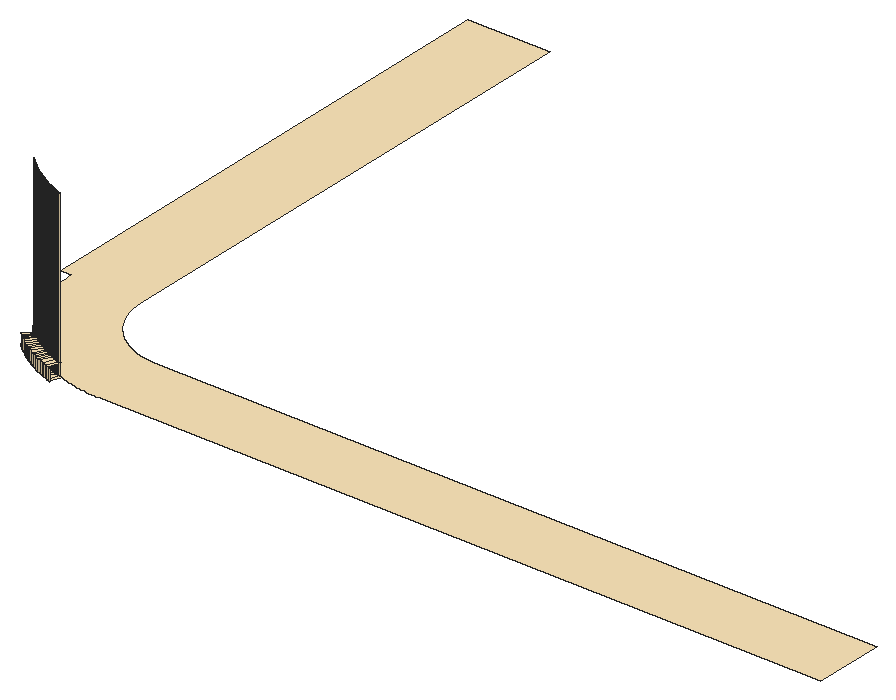
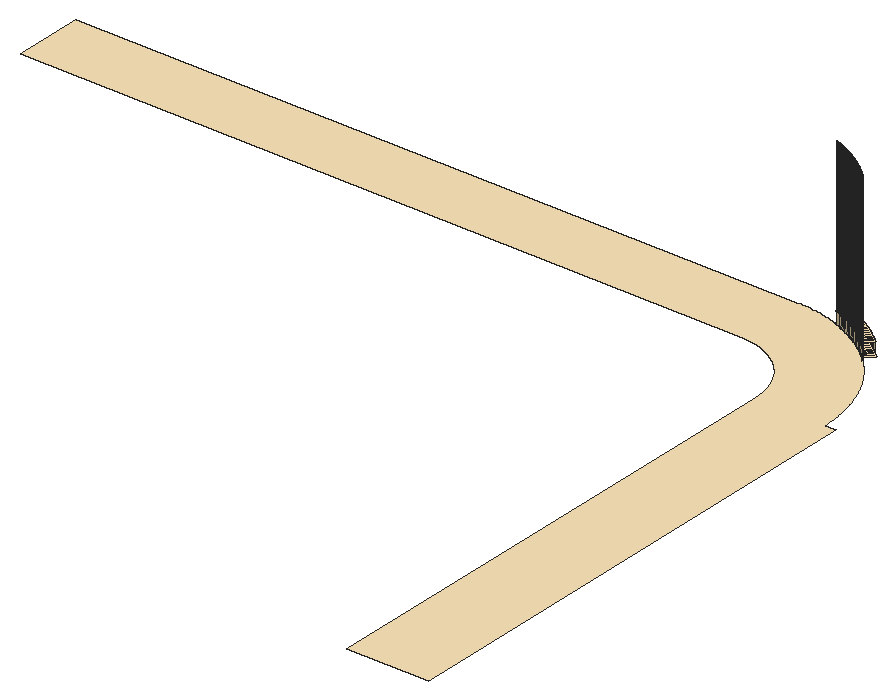
# SketchUp Ruby script. Lengths in inches.
U = 1.inch
M = Sketchup.active_model
def pt(a) = Geom::Point3d.new(a.map { |v| v * U })
def face(e, loops, mat)
  f = e.add_face(loops[0].map { |a| pt(a) })
  loops[1..].each { |l| e.add_face(l.map { |a| pt(a) }).erase! }
  f.material = f.back_material = mat if mat
  f
end
# faces: each face lists its corners as indices into pts; further lists are holes
def faces(e, pts, list, mat = nil) = list.each { |f| face(e, (f[0].is_a?(Array) ? f : [f]).map { |l| l.map { |i| pts[i] } }, mat) }
# xy, xz, yz: faces in a plane at the given z, y or x. An outline is a flat list of corners, or four numbers for a rectangle; further outlines are holes
def ring(l) = l.size == 4 ? [[l[0], l[1]], [l[2], l[1]], [l[2], l[3]], [l[0], l[3]]] : l.each_slice(2).to_a
def flat(e, list, mat, &to3) = list.each { |f| face(e, (f[0].is_a?(Array) ? f : [f]).map { |l| ring(l).map { |u, v| to3.(u, v) } }, mat) }
def xy(e, z, list, mat = nil) = flat(e, list, mat) { |x, y| [x, y, z] }
def xz(e, y, list, mat = nil) = flat(e, list, mat) { |x, z| [x, y, z] }
def yz(e, x, list, mat = nil) = flat(e, list, mat) { |y, z| [x, y, z] }
def lines(e, pts, list) = list.each { |a, b| e.add_line(pt(pts[a]), pt(pts[b])) }
# prism: a flat outline (further loops are holes) pulled along v
def prism(e, loops, v, mat = nil)
  f = face(e, loops, mat); d = Geom::Vector3d.new(v.map { |x| x * U })
  f.pushpull(f.normal.samedirection?(d) ? d.length : -d.length)
end
def box(e, o, s, mat = nil) = prism(e, [[o, [o[0] + s[0], o[1], o[2]], [o[0] + s[0], o[1] + s[1], o[2]], [o[0], o[1] + s[1], o[2]]]], [0, 0, s[2]], mat)
def at(x, y, z, deg = 0) = Geom::Transformation.translation(pt([x, y, z])) * Geom::Transformation.rotation(ORIGIN, Z_AXIS, deg.degrees)
def axes(o, x, y, z) = Geom::Transformation.new([*x, 0, *y, 0, *z, 0, *pt(o).to_a, 1])
def part(name) = M.definitions.add(name)
# library, detail: a bought-in or finely detailed component or shape, given as its bounding box
def library(name, o, s) = part(name).tap { |d| box(d.entities, o, s) }
def detail(e, o, s) = box(e.add_group.entities, o, s)
def put(e, d, t, mat = nil) = e.add_instance(d, t).tap { |i| i.material = mat if mat }
def group(e, t, mat = nil) = e.add_group.tap { |g| g.transformation = t; g.material = mat if mat }.entities
root = M.entities
M.materials.add("1026 AP 7946 SUNNY SIDE UP").color = [254, 231, 186]
xy(root,246,[[21.77,214.44,21.52,214.53,21.29,214.61,21.93,216.4,22.03,216.36,22.11,216.33,22.12,216.33,22.14,216.32,22.28,216.28,22.34,216.25,22.36,216.25,22.38,216.24],[21.29,214.61,20.92,214.75,20.53,214.9,21.23,216.66,21.25,216.65,21.33,216.62,21.4,216.59,21.43,216.58,21.47,216.57,21.5625,216.53,21.63,216.51,21.66,216.49,21.69,216.48,21.79,216.45,21.87,216.42,21.91,216.4,21.93,216.4],[20.53,214.9,20.18,215.04,19.99,215.12,20.72,216.87,20.75,216.85,20.82,216.83,20.88,216.8,21.03,216.74,21.1,216.71,21.17,216.69,21.23,216.66],[29.53,215.1,29.25,215.11,29.0625,215.12,28.75,215.13,28.5,215.15,28.25,215.16,28.0625,215.18,27.66,215.21,27.2,215.26,26.76,215.32,26.52,215.36,26.27,215.39,25.79,215.47,25.32,215.5625,24.89,215.65,24.61,215.72,24.26,215.8,24.07,215.85,23.79,215.92,23.5625,215.99,23.1875,216.09,22.86,216.19,22.63,216.27,22.41,216.34,22.17,216.42,21.97,216.49,21.62,216.62,21.27,216.76,20.9375,216.89,20.76,216.96,20.3,217.16,19.85,217.37,19.4,217.59,18.96,217.81,18.74,217.93,18.45,218.09,18.23,218.21,17.87,218.42,17.49,218.65,17.35,218.74,16.99,218.97,16.6,219.22,16.4,219.36,16.18,219.52,15.99,219.65,15.8,219.79,15.39,220.1,15.22,220.24,14.94,220.46,14.7,220.66,14.57,220.77,14.17,221.12,13.82,221.43,13.68,221.56,13.32,221.91,13.14,222.08,12.92,222.3125,12.74,222.5,12.5,222.76,12.28,222.99,12.03,223.28,11.79,223.55,11.67,223.69,11.43,224,10.99,224.55,10.86,224.72,10.71,224.93,10.43,225.32,10.16,225.72,9.9,226.13,9.77,226.33,9.55,226.68,9.43,226.88,9.32,227.09,9.2,227.29,9.1,227.47,8.98,227.7,8.76,228.12,8.65,228.34,8.45,228.75,8.24,229.21,8.16,229.38,8.04,229.65,7.89,230.03,7.8,230.25,7.72,230.47,7.6,230.79,7.49,231.1,7.41,231.33,7.33,231.57,7.26,231.79,7.1875,232.02,7.12,232.24,6.98,232.73,6.79,233.49,6.72,233.83,6.63,234.23,6.58,234.52,6.53,234.75,6.5,234.96,6.46,235.21,6.42,235.45,6.35,235.93,6.27,236.65,6.25,236.89,6.22,237.3,6.19,237.77,6.18,238,6.17,238.47,6.16,238.79,6.16,238.9375,6,238.9375,4.16,238.95,4,326,18,326,18,238.75,18.01,238.625,18.01,238.5,18.02,238.37,18.02,238.25,18.03,238.12,18.04,238,18.05,237.87,18.07,237.75,18.08,237.62,18.09,237.5,18.11,237.37,18.13,237.25,18.15,237.12,18.17,237,18.21,236.75,18.24,236.63,18.26,236.51,18.29,236.38,18.38,236.02,18.41,235.89,18.44,235.77,18.48,235.65,18.51,235.53,18.59,235.29,18.625,235.17,18.67,235.05,18.71,234.94,18.75,234.82,18.8,234.7,18.84,234.58,18.89,234.47,18.9375,234.35,18.99,234.23,19.04,234.12,19.09,234,19.14,233.89,19.2,233.78,19.25,233.66,19.37,233.44,19.42,233.33,19.48,233.22,19.55,233.11,19.67,232.89,19.74,232.78,19.8,232.68,19.87,232.57,19.9375,232.46,20,232.36,20.08,232.25,20.29,231.95,20.37,231.85,20.44,231.74,20.52,231.65,20.6,231.55,20.67,231.45,20.83,231.25,20.92,231.16,21,231.0625,21.08,230.97,21.17,230.88,21.25,230.79,21.34,230.69,21.43,230.6,21.51,230.51,21.6,230.43,21.69,230.34,21.79,230.25,21.88,230.17,21.97,230.08,22.0625,230,22.16,229.92,22.25,229.83,22.45,229.67,22.55,229.6,22.65,229.52,22.74,229.44,22.85,229.37,22.95,229.29,23.25,229.08,23.36,229,23.46,228.9375,23.57,228.87,23.68,228.8,23.78,228.74,23.89,228.67,24.11,228.55,24.22,228.48,24.33,228.42,24.44,228.37,24.66,228.25,24.78,228.2,24.89,228.14,25,228.09,25.12,228.04,25.23,227.99,25.35,227.9375,25.47,227.89,25.58,227.84,25.7,227.8,25.82,227.75,25.94,227.71,26.05,227.67,26.17,227.625,26.29,227.59,26.53,227.51,26.65,227.48,26.77,227.44,26.89,227.41,27.02,227.38,27.38,227.29,27.51,227.26,27.63,227.24,27.75,227.21,28,227.17,28.12,227.15,28.25,227.13,28.37,227.11,28.5,227.09,28.62,227.08,28.75,227.07,28.87,227.05,29,227.04,29.12,227.03,29.25,227.02,29.37,227.02,29.5,227.01,29.625,227.01,29.65,227,153,227,153,215.1],[19.99,215.12,19.74,215.22,19.49,215.34,20.26,217.06,20.3,217.05,20.38,217.01,20.43,216.99,20.47,216.97,20.53,216.95,20.6,216.92,20.65,216.9,20.7,216.875,20.72,216.87],
  [19.49,215.34,19,215.56,19.81,217.27,19.95,217.2,20.01,217.18,20.08,217.15,20.17,217.11,20.2,217.09,20.26,217.06],[19,215.56,18.52,215.79,19.35,217.49,19.39,217.47,19.53,217.41,19.55,217.39,19.63,217.36,19.74,217.3,19.78,217.28,19.81,217.27],[18.52,215.79,18.27,215.92,18.04,216.04,18.91,217.71,19.1,217.62,19.31,217.51,19.32,217.51,19.33,217.5,19.35,217.49],[18.04,216.04,17.79,216.17,18.68,217.83,18.6875,217.83,18.82,217.77,18.88,217.73,18.89,217.73,18.89,217.72,18.91,217.71],[17.79,216.17,17.48,216.34,17.24,216.47,18.18,218.11,18.24,218.08,18.27,218.06,18.37,218.01,18.4375,217.97,18.46,217.96,18.48,217.95,18.59,217.89,18.66,217.85,18.68,217.83],
  [21.91,216.4,21.87,216.42,21.79,216.45,21.69,216.48,21.66,216.49,21.63,216.51,21.5625,216.53,21.47,216.57,21.43,216.58,21.4,216.59,21.33,216.62,21.25,216.65,21.23,216.66,21.27,216.76,21.62,216.62,21.97,216.49,21.93,216.4],[17.24,216.47,16.85,216.7,17.81,218.33,17.82,218.32,17.86,218.29,17.9375,218.25,18,218.22,18.03,218.2,18.07,218.18,18.15,218.13,18.18,218.11],[21.23,216.66,21.17,216.69,21.1,216.71,21.03,216.74,20.88,216.8,20.82,216.83,20.75,216.85,20.72,216.87,20.76,216.96,20.9375,216.89,21.27,216.76],[16.85,216.7,16.44,216.94,16.28,217.04,17.29,218.64,17.31,218.63,17.35,218.6,17.4,218.57,17.46,218.54,17.52,218.5,17.57,218.47,17.61,218.44,17.66,218.41,17.73,218.375,17.78,218.34,17.81,218.33],[20.72,216.87,20.7,216.875,20.65,216.9,20.6,216.92,20.53,216.95,20.47,216.97,20.43,216.99,20.38,217.01,20.3,217.05,20.26,217.06,20.3,217.16,20.76,216.96],
  [16.28,217.04,15.89,217.29,16.93,218.875,16.93,218.87,16.99,218.83,17.0625,218.79,17.1,218.76,17.14,218.74,17.29,218.64],[20.26,217.06,20.2,217.09,20.17,217.11,20.08,217.15,20.01,217.18,19.95,217.2,19.81,217.27,19.85,217.37,20.3,217.16],[19.81,217.27,19.78,217.28,19.74,217.3,19.63,217.36,19.55,217.39,19.53,217.41,19.39,217.47,19.35,217.49,19.4,217.59,19.85,217.37],[15.89,217.29,15.48,217.56,16.54,219.13,16.58,219.11,16.67,219.04,16.69,219.03,16.78,218.97,16.86,218.91,16.93,218.875],[19.35,217.49,19.33,217.5,19.32,217.51,19.31,217.51,19.1,217.62,18.91,217.71,18.96,217.81,19.4,217.59],
  [15.48,217.56,15.25,217.72,15.02,217.89,16.11,219.43,16.16,219.39,16.28,219.31,16.3,219.29,16.37,219.25,16.47,219.18,16.49,219.16,16.51,219.15,16.54,219.13],[18.91,217.71,18.89,217.72,18.89,217.73,18.88,217.73,18.82,217.77,18.6875,217.83,18.68,217.83,18.74,217.93,18.96,217.81],[18.68,217.83,18.66,217.85,18.59,217.89,18.48,217.95,18.46,217.96,18.4375,217.97,18.37,218.01,18.27,218.06,18.24,218.08,18.18,218.11,18.23,218.21,18.45,218.09,18.74,217.93],[15.02,217.89,14.8125,218.03,14.6,218.1875,15.73,219.7,15.89,219.58,16.08,219.45,16.09,219.44,16.1,219.4375,16.11,219.43],[18.18,218.11,18.15,218.13,18.07,218.18,18.03,218.2,18,218.22,17.9375,218.25,17.86,218.29,17.82,218.32,17.81,218.33,17.87,218.42,18.23,218.21],
  [14.6,218.1875,14.17,218.52,15.32,220.01,15.33,220.01,15.42,219.93,15.49,219.88,15.5,219.875,15.51,219.86,15.63,219.78,15.69,219.73,15.7,219.73,15.7,219.72,15.73,219.7],[17.81,218.33,17.78,218.34,17.73,218.375,17.66,218.41,17.61,218.44,17.57,218.47,17.52,218.5,17.46,218.54,17.4,218.57,17.35,218.6,17.31,218.63,17.29,218.64,17.35,218.74,17.49,218.65,17.87,218.42],[14.17,218.52,13.97,218.67,15.15,220.15,15.23,220.09,15.29,220.04,15.32,220.01],[17.29,218.64,17.14,218.74,17.1,218.76,17.0625,218.79,16.99,218.83,16.93,218.87,16.93,218.875,16.99,218.97,17.35,218.74],[13.97,218.67,13.68,218.91,14.87,220.37,14.93,220.33,14.96,220.3,15.03,220.24,15.09,220.19,15.12,220.17,15.14,220.15,15.15,220.15],
  [16.93,218.875,16.86,218.91,16.78,218.97,16.69,219.03,16.67,219.04,16.58,219.11,16.54,219.13,16.6,219.22,16.99,218.97],[13.68,218.91,13.42,219.125,14.625,220.57,14.7,220.51,14.74,220.48,14.77,220.45,14.84,220.39,14.87,220.37],[13.42,219.125,13.27,219.25,14.5,220.68,14.51,220.67,14.55,220.64,14.59,220.6,14.625,220.57],[16.54,219.13,16.51,219.15,16.49,219.16,16.47,219.18,16.37,219.25,16.3,219.29,16.28,219.31,16.16,219.39,16.11,219.43,16.18,219.52,16.4,219.36,16.6,219.22],[13.27,219.25,12.84,219.62,14.09,221.03,14.1,221.03,14.23,220.9,14.28,220.87,14.36,220.79,14.46,220.71,14.5,220.68],
  [16.11,219.43,16.1,219.4375,16.09,219.44,16.08,219.45,15.89,219.58,15.73,219.7,15.8,219.79,15.99,219.65,16.18,219.52],[12.84,219.62,12.47,219.96,13.74,221.35,13.75,221.33,13.8125,221.28,13.88,221.22,13.94,221.16,13.99,221.12,14.06,221.06,14.09,221.03],[15.73,219.7,15.7,219.72,15.7,219.73,15.69,219.73,15.63,219.78,15.51,219.86,15.5,219.875,15.49,219.88,15.42,219.93,15.33,220.01,15.32,220.01,15.39,220.1,15.8,219.79],[15.32,220.01,15.29,220.04,15.23,220.09,15.15,220.15,15.22,220.24,15.39,220.1],[15.14,220.15,15.12,220.17,15.09,220.19,15.03,220.24,14.96,220.3,14.93,220.33,14.87,220.37,14.94,220.46,15.22,220.24,15.15,220.15],
  [14.87,220.37,14.84,220.39,14.77,220.45,14.74,220.48,14.7,220.51,14.625,220.57,14.7,220.66,14.94,220.46],[14.625,220.57,14.59,220.6,14.55,220.64,14.51,220.67,14.5,220.68,14.57,220.77,14.7,220.66],[14.5,220.68,14.46,220.71,14.36,220.79,14.28,220.87,14.23,220.9,14.1,221.03,14.09,221.03,14.17,221.12,14.57,220.77],[14.09,221.03,14.06,221.06,13.99,221.12,13.94,221.16,13.88,221.22,13.8125,221.28,13.75,221.33,13.74,221.35,13.82,221.43,14.17,221.12],[13.73,221.35,13.71,221.375,13.63,221.45,13.6,221.48,13.68,221.56,13.82,221.43,13.74,221.35],
  [13.6,221.48,13.57,221.5,13.55,221.52,13.54,221.54,13.45,221.62,13.39,221.68,13.38,221.6875,13.37,221.7,13.26,221.8,13.24,221.82,13.32,221.91,13.68,221.56]],"1026 AP 7946 SUNNY SIDE UP")
xy(root,248,[[21.52,214.53,22.17,216.42,21.97,216.49,21.62,216.62,20.92,214.75,21.29,214.61],[20.92,214.75,21.62,216.62,21.27,216.76,20.9375,216.89,20.18,215.04,20.53,214.9],[20.18,215.04,20.9375,216.89,20.76,216.96,20.3,217.16,19.49,215.34,19.74,215.22,19.99,215.12],[19.49,215.34,20.3,217.16,19.85,217.37,19,215.56],[19,215.56,19.85,217.37,19.4,217.59,18.52,215.79],
  [18.52,215.79,19.4,217.59,19.18,217.7,18.27,215.92],[18.27,215.92,19.18,217.7,18.96,217.81,18.74,217.93,17.79,216.17,18.04,216.04],[17.79,216.17,18.74,217.93,18.45,218.09,17.48,216.34],[17.48,216.34,18.45,218.09,18.23,218.21,17.87,218.42,16.85,216.7,17.24,216.47],[16.85,216.7,17.87,218.42,17.49,218.65,17.35,218.74,16.28,217.04,16.44,216.94],
  [16.28,217.04,17.35,218.74,16.99,218.97,15.89,217.29],[15.89,217.29,16.99,218.97,16.6,219.22,15.48,217.56],[15.48,217.56,16.6,219.22,16.4,219.36,16.18,219.52,15.02,217.89,15.25,217.72],[15.02,217.89,16.18,219.52,15.99,219.65,15.8,219.79,14.6,218.1875,14.8125,218.03],[14.6,218.1875,15.8,219.79,15.39,220.1,14.17,218.52],
  [14.17,218.52,15.39,220.1,15.22,220.24,13.97,218.67],[13.97,218.67,15.22,220.24,14.94,220.46,13.68,218.91],[13.68,218.91,14.94,220.46,14.7,220.66,13.42,219.125],[13.42,219.125,14.7,220.66,14.57,220.77,13.27,219.25],[13.27,219.25,14.57,220.77,14.17,221.12,12.84,219.62]],"1026 AP 7946 SUNNY SIDE UP")
xz(root,217.51,[[19.31,246,19.32,274]],"1026 AP 7946 SUNNY SIDE UP")
xz(root,217.73,[[18.88,246,18.89,274]],"1026 AP 7946 SUNNY SIDE UP")
xz(root,219.73,[[15.69,246,15.7,274]],"1026 AP 7946 SUNNY SIDE UP")
yz(root,15.7,[[219.72,246,219.73,274]],"1026 AP 7946 SUNNY SIDE UP")
yz(root,18.89,[[217.72,246,217.73,274]],"1026 AP 7946 SUNNY SIDE UP")
p = [[21.77,214.44,246],[21.77,214.44,248],[21.52,214.53,248],[21.52,214.53,246],[22.02,214.36,246],[22.02,214.36,248],
  [21.29,214.61,248],[21.29,214.61,246],[20.92,214.75,248],[20.92,214.75,246],[20.53,214.9,248],[20.53,214.9,246],
  [20.18,215.04,248],[20.18,215.04,246],[19.99,215.12,248],[19.99,215.12,246],[19.74,215.22,248],[19.74,215.22,246],
  [19.49,215.34,248],[19.49,215.34,246],[19,215.56,248],[19,215.56,246],[18.52,215.79,248],[18.52,215.79,246],
  [18.27,215.92,248],[18.27,215.92,246],[18.04,216.04,248],[18.04,216.04,246],[17.79,216.17,248],[17.79,216.17,246],
  [17.48,216.34,248],[17.48,216.34,246],[17.24,216.47,248],[17.24,216.47,246],[22.03,216.36,246],[22.11,216.33,246],
  [22.11,216.33,274],[22.03,216.36,274],[21.69,216.48,246],[21.79,216.45,246],[21.79,216.45,274],[21.69,216.48,274],
  [21.87,216.42,246],[21.87,216.42,274],[21.89,216.41,246],[21.89,216.41,274],[21.91,216.4,246],[21.91,216.4,274],
  [21.93,216.4,246],[16.85,216.7,248],[16.85,216.7,246],[21.47,216.57,246],[21.5625,216.53,246],[21.5625,216.53,274],
  [21.47,216.57,274],[21.63,216.51,246],[21.63,216.51,274],[21.66,216.49,246],[21.66,216.49,274],[21.97,216.49,248],
  [21.97,216.49,246],[21.62,216.62,246],[21.62,216.62,248],[21.25,216.65,246],[21.33,216.62,246],[21.33,216.62,274],
  [21.25,216.65,274],[21.4,216.59,246],[21.4,216.59,274],[21.27,216.76,246],[21.27,216.76,248],[21.43,216.58,246],
  [21.43,216.58,274],[16.44,216.94,248],[16.44,216.94,246],[20.98,216.76,246],[21.03,216.74,246],[21.03,216.74,274],
  [20.98,216.76,274],[21.1,216.71,246],[21.1,216.71,274],[21.17,216.69,246],[21.17,216.69,274],[21.21,216.67,246],
  [21.21,216.67,274],[21.23,216.66,246],[20.75,216.85,246],[20.82,216.83,246],[20.82,216.83,274],[20.75,216.85,274],
  [20.88,216.8,246],[20.88,216.8,274],[20.93,216.78,246],[20.93,216.78,274],[20.9375,216.89,246],[20.9375,216.89,248],
  [16.28,217.04,248],[16.28,217.04,246],[20.47,216.97,246],[20.53,216.95,246],[20.53,216.95,274],[20.47,216.97,274],
  [20.6,216.92,246],[20.6,216.92,274],[20.65,216.9,246],[20.65,216.9,274],[20.7,216.875,246],[20.7,216.875,274],
  [20.72,216.87,246],[20.76,216.96,246],[20.76,216.96,248],[15.89,217.29,248],[15.89,217.29,246],[20.24,217.07,246],
  [20.26,217.06,246],[20.3,217.05,246],[20.3,217.05,274],[20.24,217.07,274],[20.38,217.01,246],[20.38,217.01,274],
  [20.43,216.99,246],[20.43,216.99,274],[20.53,217.06,246],[20.53,217.06,248],[20.01,217.18,246],[20.08,217.15,246],
  [20.08,217.15,274],[20.01,217.18,274],[20.17,217.11,246],[20.17,217.11,274],[20.2,217.09,246],[20.2,217.09,274],
  [20.3,217.16,246],[20.3,217.16,248],[19.85,217.25,246],[19.95,217.2,246],[19.95,217.2,274],[19.85,217.25,274],
  [19.85,217.37,246],[19.85,217.37,248],[19.98,217.19,246],[19.98,217.19,274],[15.48,217.56,248],[15.48,217.56,246],
  [19.63,217.36,246],[19.74,217.3,246],[19.74,217.3,274],[19.63,217.36,274],[19.76,217.29,246],[19.76,217.29,274],
  [19.78,217.28,246],[19.78,217.28,274],[19.81,217.27,246],[19.39,217.47,246],[19.53,217.41,246],[19.53,217.41,274],
  [19.39,217.47,274],[19.4,217.59,246],[19.4,217.59,248],[19.54,217.4,246],[19.54,217.4,274],[19.55,217.39,246],
  [19.55,217.39,274],[19.1,217.62,246],[19.31,217.51,246],[19.31,217.51,274],[19.1,217.62,274],[19.32,217.51,246],
  [19.33,217.5,246],[19.33,217.5,274],[19.32,217.51,274],[19.35,217.49,246],[15.25,217.72,248],[15.25,217.72,246],
  [18.89,217.72,246],[18.91,217.71,246],[18.89,217.72,274],[19.18,217.7,246],[19.18,217.7,248],[15.02,217.89,248],
  [15.02,217.89,246],[18.82,217.77,246],[18.88,217.73,246],[18.88,217.73,274],[18.82,217.77,274],[18.96,217.81,246],
  [18.96,217.81,248],[18.59,217.89,246],[18.66,217.85,246],[18.66,217.85,274],[18.59,217.89,274],[18.67,217.84,246],
  [18.67,217.84,274],[18.68,217.83,246],[18.6875,217.83,246],[18.6875,217.83,274],[18.74,217.93,246],[18.74,217.93,248],
  [14.8125,218.03,248],[14.8125,218.03,246],[18.45,218.09,246],[18.45,218.09,248],[18.46,217.96,246],[18.48,217.95,246],
  [18.48,217.95,274],[18.46,217.96,274],[14.6,218.1875,248],[14.6,218.1875,246],[18.27,218.06,246],[18.37,218.01,246],
  [18.37,218.01,274],[18.27,218.06,274],[18.4375,217.97,246],[18.4375,217.97,274],[18.07,218.18,246],[18.15,218.13,246],
  [18.15,218.13,274],[18.07,218.18,274],[18.18,218.11,246],[18.22,218.09,246],[18.22,218.09,274],[18.24,218.08,246],
  [18.24,218.08,274],[18.23,218.21,246],[18.23,218.21,248],[14.17,218.52,248],[14.17,218.52,246],[17.9375,218.25,246],
  [18,218.22,246],[18,218.22,274],[17.9375,218.25,274],[17.87,218.42,246],[17.87,218.42,248],[18.03,218.2,246],
  [18.03,218.2,274],[17.73,218.375,246],[17.78,218.34,246],[17.78,218.34,274],[17.73,218.375,274],[17.81,218.33,246],
  [17.82,218.32,246],[17.82,218.32,274],[17.86,218.29,246],[17.86,218.29,274],[17.49,218.65,246],[17.49,218.65,248],
  [17.57,218.47,246],[17.61,218.44,246],[17.61,218.44,274],[17.57,218.47,274],[17.66,218.41,246],[17.66,218.41,274],
  [13.97,218.67,248],[13.97,218.67,246],[17.4,218.57,246],[17.46,218.54,246],[17.46,218.54,274],[17.4,218.57,274],
  [17.52,218.5,246],[17.52,218.5,274],[17.26,218.66,246],[17.29,218.64,246],[17.31,218.63,246],[17.31,218.63,274],
  [17.26,218.66,274],[17.35,218.6,246],[17.35,218.6,274],[17.35,218.74,246],[17.35,218.74,248],[13.68,218.91,248],
  [13.68,218.91,246],[16.99,218.97,246],[16.99,218.97,248],[17.1,218.76,246],[17.14,218.74,246],[17.14,218.74,274],
  [17.1,218.76,274],[17.2,218.7,246],[17.2,218.7,274],[16.93,218.87,246],[16.99,218.83,246],[16.99,218.83,274],
  [16.93,218.87,274],[17.0625,218.79,246],[17.0625,218.79,274],[13.42,219.125,248],[13.42,219.125,246],[16.78,218.97,246],
  [16.86,218.91,246],[16.86,218.91,274],[16.78,218.97,274],[16.9,218.89,246],[16.9,218.89,274],[16.93,218.875,246],
  [16.58,219.11,246],[16.67,219.04,246],[16.67,219.04,274],[16.58,219.11,274],[16.6,219.22,246],[16.6,219.22,248],
  [16.69,219.03,246],[16.69,219.03,274],[16.72,219.01,246],[16.72,219.01,274],[13.27,219.25,248],[13.27,219.25,246],
  [16.51,219.15,246],[16.54,219.13,246],[16.51,219.15,274],[16.3,219.29,246],[16.37,219.25,246],[16.37,219.25,274],
  [16.3,219.29,274],[16.47,219.18,246],[16.47,219.18,274],[16.4,219.36,246],[16.4,219.36,248],[16.49,219.16,246],
  [16.49,219.16,274],[16.16,219.39,246],[16.28,219.31,246],[16.28,219.31,274],[16.16,219.39,274],[16.29,219.3,246],
  [16.29,219.3,274],[15.89,219.58,246],[16.08,219.45,246],[16.08,219.45,274],[15.89,219.58,274],[16.09,219.44,246],
  [16.09,219.44,274],[16.1,219.4375,246],[16.1,219.4375,274],[16.11,219.43,246],[16.18,219.52,246],[16.18,219.52,248],
  [15.99,219.65,246],[15.99,219.65,248],[15.7,219.72,246],[15.73,219.7,246],[15.7,219.72,274],[15.63,219.78,246],
  [15.69,219.73,246],[15.69,219.73,274],[15.63,219.78,274],[15.8,219.79,246],[15.8,219.79,248],[15.39,220.1,246],
  [15.39,220.1,248],[15.51,219.86,246],[15.51,219.86,274],[15.33,220.01,246],[15.42,219.93,246],[15.42,219.93,274],
  [15.33,220.01,274],[15.49,219.88,246],[15.49,219.88,274],[15.5,219.875,246],[15.5,219.875,274],[15.23,220.09,246],
  [15.29,220.04,246],[15.29,220.04,274],[15.23,220.09,274],[15.31,220.02,246],[15.31,220.02,274],[15.32,220.01,246],
  [15.14,220.15,246],[15.15,220.15,246],[15.14,220.15,274],[15.22,220.24,246],[15.22,220.24,248],[14.94,220.46,246],
  [14.94,220.46,248],[14.96,220.3,246],[15.03,220.24,246],[15.03,220.24,274],[14.96,220.3,274],[15.09,220.19,246],
  [15.09,220.19,274],[15.12,220.17,246],[15.12,220.17,274],[14.84,220.39,246],[14.87,220.37,246],[14.9,220.35,246],
  [14.9,220.35,274],[14.84,220.39,274],[14.93,220.33,246],[14.93,220.33,274],[14.74,220.48,246],[14.77,220.45,246],
  [14.77,220.45,274],[14.74,220.48,274],[14.59,220.6,246],[14.625,220.57,246],[14.65,220.55,246],[14.65,220.55,274],
  [14.59,220.6,274],[14.7,220.51,246],[14.7,220.51,274],[14.7,220.66,246],[14.7,220.66,248],[14.51,220.67,246],
  [14.55,220.64,246],[14.55,220.64,274],[14.51,220.67,274],[14.41,220.75,246],[14.46,220.71,246],[14.46,220.71,274],
  [14.41,220.75,274],[14.5,220.68,246],[14.57,220.77,246],[14.57,220.77,248],[14.17,221.12,246],[14.17,221.12,248],
  [14.28,220.87,246],[14.32,220.83,246],[14.32,220.83,274],[14.28,220.87,274],[14.36,220.79,246],[14.36,220.79,274],
  [14.18,220.95,246],[14.23,220.9,246],[14.23,220.9,274],[14.18,220.95,274],[14.06,221.06,246],[14.09,221.03,246],
  [14.1,221.03,246],[14.1,221.03,274],[14.06,221.06,274],[14.13,221,246],[14.13,221,274],[13.82,221.43,246],
  [13.82,221.43,248],[13.94,221.16,246],[13.99,221.12,246],[13.99,221.12,274],[13.94,221.16,274],[13.8125,221.28,246],
  [13.88,221.22,246],[13.88,221.22,274],[13.8125,221.28,274],[13.91,221.19,246],[13.91,221.19,274],[13.73,221.35,246],
  [13.74,221.35,246],[13.75,221.33,246],[13.75,221.33,274],[13.73,221.35,274],[13.57,221.5,246],[13.6,221.48,246],
  [13.63,221.45,246],[13.63,221.45,274],[13.57,221.5,274],[13.71,221.375,246],[13.71,221.375,274],[13.68,221.56,246],
  [13.68,221.56,248],[13.45,221.62,246],[13.54,221.54,246],[13.54,221.54,274],[13.45,221.62,274],[13.55,221.52,246],
  [13.55,221.52,274],[13.32,221.91,246],[13.32,221.91,248],[13.39,221.68,246],[13.39,221.68,274],[13.37,221.7,246],
  [13.38,221.6875,246],[13.38,221.6875,274],[13.37,221.7,274]]
faces(root,p,[[0,1,2,3],[4,5,1,0],[3,2,6,7],[7,6,8,9],[9,8,10,11],[11,10,12,13],[13,12,14,15],[15,14,16,17],
  [17,16,18,19],[19,18,20,21],[21,20,22,23],[23,22,24,25],[25,24,26,27],[27,26,28,29],[29,28,30,31],[31,30,32,33],
  [34,35,36,37],[38,39,40,41],[39,42,43,40],[42,44,45,43],[44,46,47,45],[46,48,34,37,47],[33,32,49,50],[51,52,53,54],
  [52,55,56,53],[55,57,58,56],[59,60,61,62],[57,38,41,58],[63,64,65,66],[64,67,68,65],[62,61,69,70],[67,71,72,68],
  [71,51,54,72],[50,49,73,74],[75,76,77,78],[76,79,80,77],[79,81,82,80],[81,83,84,82],[83,85,63,66,84],[86,87,88,89],
  [87,90,91,88],[90,92,93,91],[92,75,78,93],[70,69,94,95],[74,73,96,97],[98,99,100,101],[99,102,103,100],[102,104,105,103],
  [104,106,107,105],[106,108,86,89,107],[95,94,109,110],[97,96,111,112],[113,114,115,116,117],[115,118,119,116],[118,120,121,119],[120,98,101,121],
  [110,109,122,123],[124,125,126,127],[125,128,129,126],[128,130,131,129],[130,113,117,131],[123,122,132,133],[134,135,136,137],[133,132,138,139],
  [135,140,141,136],[140,124,127,141],[112,111,142,143],[144,145,146,147],[145,148,149,146],[148,150,151,149],[150,152,134,137,151],[153,154,155,156],
  [139,138,157,158],[154,159,160,155],[159,161,162,160],[161,144,147,162],[163,164,165,166],[167,168,169,170],[168,171,153,156,169],[143,142,172,173],
  [174,175,163,166,176],[158,157,177,178],[173,172,179,180],[181,182,183,184],[178,177,185,186],[187,188,189,190],[188,191,192,189],[191,193,194,195,192],
  [194,181,184,195],[186,185,196,197],[180,179,198,199],[197,196,200,201],[202,203,204,205],[203,187,190,204],[199,198,206,207],[208,209,210,211],
  [209,212,213,210],[212,202,205,213],[214,215,216,217],[215,218,219,220,216],[219,221,222,220],[221,208,211,222],[201,200,223,224],[207,206,225,226],
  [227,228,229,230],[224,223,231,232],[228,233,234,229],[233,214,217,234],[235,236,237,238],[236,239,240,241,237],[240,242,243,241],[242,227,230,243],
  [232,231,244,245],[246,247,248,249],[247,250,251,248],[250,235,238,251],[226,225,252,253],[254,255,256,257],[255,258,259,256],[258,246,249,259],
  [260,261,262,263,264],[262,265,266,263],[245,244,267,268],[265,254,257,266],[253,252,269,270],[268,267,271,272],[273,274,275,276],[274,277,278,275],
  [277,260,264,278],[279,280,281,282],[280,283,284,281],[283,273,276,284],[270,269,285,286],[287,288,289,290],[288,291,292,289],[291,293,279,282,292],
  [294,295,296,297],[272,271,298,299],[295,300,301,296],[300,302,303,301],[302,287,290,303],[286,285,304,305],[306,307,294,297,308],[309,310,311,312],
  [310,313,314,311],[299,298,315,316],[313,317,318,314],[317,306,308,318],[319,320,321,322],[320,323,324,321],[323,309,312,324],[325,326,327,328],
  [326,329,330,327],[329,331,332,330],[331,333,319,322,332],[316,315,334,335],[335,334,336,337],[338,339,325,328,340],[341,342,343,344],[337,336,345,346],
  [346,345,347,348],[349,341,344,350],[351,352,353,354],[352,355,356,353],[355,357,358,356],[357,349,350,358],[359,360,361,362],[360,363,364,361],
  [363,365,351,354,364],[366,367,359,362,368],[348,347,369,370],[370,369,371,372],[373,374,375,376],[374,377,378,375],[377,379,380,378],[379,366,368,380],
  [381,382,383,384,385],[383,386,387,384],[386,373,376,387],[388,389,390,391],[389,381,385,390],[392,393,394,395,396],[394,397,398,395],[397,388,391,398],
  [372,371,399,400],[401,402,403,404],[402,392,396,403],[405,406,407,408],[406,409,401,404,407],[400,399,410,411],[411,410,412,413],[414,415,416,417],
  [415,418,419,416],[418,405,408,419],[420,421,422,423],[421,414,417,422],[424,425,426,427,428],[426,429,430,427],[429,420,423,430],[413,412,431,432],
  [433,434,435,436],[434,424,428,435],[437,438,439,440],[438,441,442,439],[441,433,436,442],[443,444,445,446,447],[445,437,440,446],[448,449,450,451,452],
  [450,453,454,451],[453,443,447,454],[432,431,455,456],[457,458,459,460],[458,461,462,459],[461,448,452,462],[456,455,463,464],[465,457,460,466],
  [467,468,469,470],[468,465,466,469]],"1026 AP 7946 SUNNY SIDE UP")
